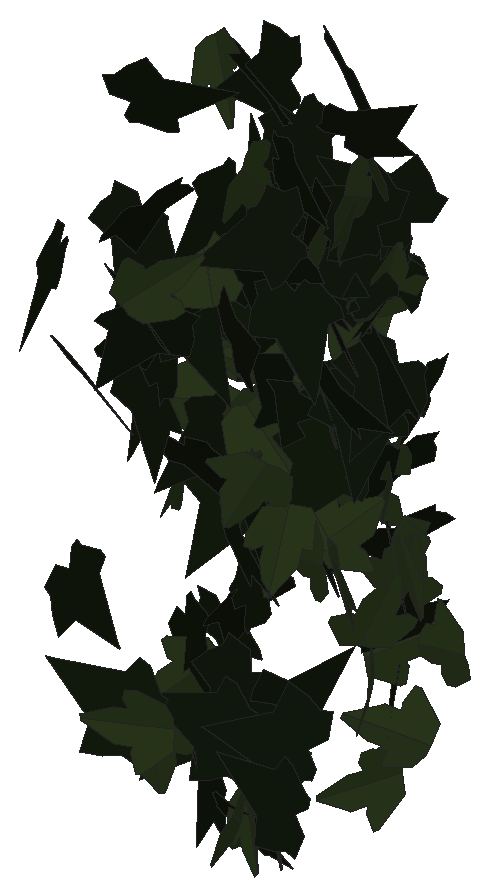
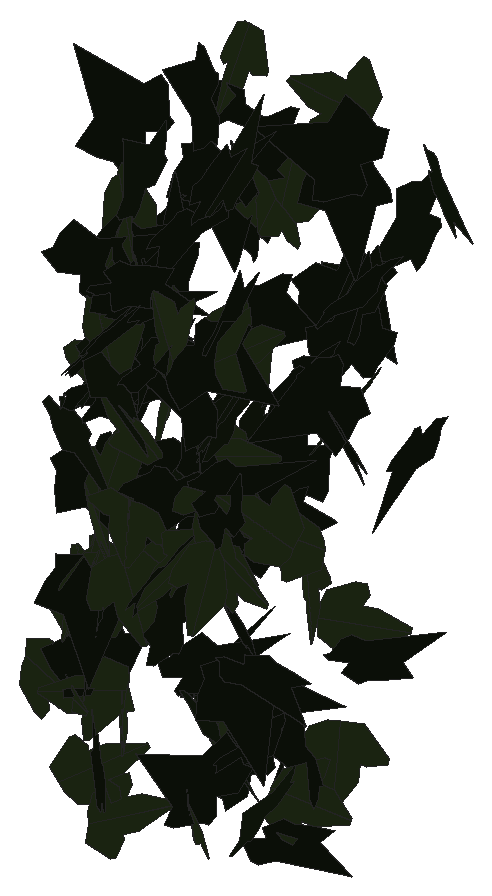
# SketchUp Ruby script. Lengths in inches.
U = 1.inch
M = Sketchup.active_model
def pt(a) = Geom::Point3d.new(a.map { |v| v * U })
def face(e, loops, mat)
  f = e.add_face(loops[0].map { |a| pt(a) })
  loops[1..].each { |l| e.add_face(l.map { |a| pt(a) }).erase! }
  f.material = f.back_material = mat if mat
  f
end
# faces: each face lists its corners as indices into pts; further lists are holes
def faces(e, pts, list, mat = nil) = list.each { |f| face(e, (f[0].is_a?(Array) ? f : [f]).map { |l| l.map { |i| pts[i] } }, mat) }
# xy, xz, yz: faces in a plane at the given z, y or x. An outline is a flat list of corners, or four numbers for a rectangle; further outlines are holes
def ring(l) = l.size == 4 ? [[l[0], l[1]], [l[2], l[1]], [l[2], l[3]], [l[0], l[3]]] : l.each_slice(2).to_a
def flat(e, list, mat, &to3) = list.each { |f| face(e, (f[0].is_a?(Array) ? f : [f]).map { |l| ring(l).map { |u, v| to3.(u, v) } }, mat) }
def xy(e, z, list, mat = nil) = flat(e, list, mat) { |x, y| [x, y, z] }
def xz(e, y, list, mat = nil) = flat(e, list, mat) { |x, z| [x, y, z] }
def yz(e, x, list, mat = nil) = flat(e, list, mat) { |y, z| [x, y, z] }
def lines(e, pts, list) = list.each { |a, b| e.add_line(pt(pts[a]), pt(pts[b])) }
# prism: a flat outline (further loops are holes) pulled along v
def prism(e, loops, v, mat = nil)
  f = face(e, loops, mat); d = Geom::Vector3d.new(v.map { |x| x * U })
  f.pushpull(f.normal.samedirection?(d) ? d.length : -d.length)
end
def box(e, o, s, mat = nil) = prism(e, [[o, [o[0] + s[0], o[1], o[2]], [o[0] + s[0], o[1] + s[1], o[2]], [o[0], o[1] + s[1], o[2]]]], [0, 0, s[2]], mat)
def at(x, y, z, deg = 0) = Geom::Transformation.translation(pt([x, y, z])) * Geom::Transformation.rotation(ORIGIN, Z_AXIS, deg.degrees)
def axes(o, x, y, z) = Geom::Transformation.new([*x, 0, *y, 0, *z, 0, *pt(o).to_a, 1])
def part(name) = M.definitions.add(name)
# library, detail: a bought-in or finely detailed component or shape, given as its bounding box
def library(name, o, s) = part(name).tap { |d| box(d.entities, o, s) }
def detail(e, o, s) = box(e.add_group.entities, o, s)
def put(e, d, t, mat = nil) = e.add_instance(d, t).tap { |i| i.material = mat if mat }
def group(e, t, mat = nil) = e.add_group.tap { |g| g.transformation = t; g.material = mat if mat }.entities
root = M.entities
M.materials.add("efeu1").color = [18, 25, 13]
M.materials.add("efeu2").color = [43, 57, 29]
c1 = part("ivyleaf_10")
p = [[0,0.5,-0.03],[-0.0625,2.02,-0.43],[-0.19,2.01,-0.46],[-0.54,1.05,-0.29],[-0.52,0.625,-0.18],[-0.83,0.76,-0.28],
  [-1.16,0.64,-0.33],[-1.15,0.33,-0.24],[-0.77,-0.39,0.02],[-0.3,-0.51,0.16],[0.04,-0.48,0.23],[-0.02,2.01,-0.4375],
  [-0.06,2.01,-0.43],[0.04,-0.49,0.23],[0.67,-0.49,0.14],[1.38,0.36,-0.2],[1.375,0.51,-0.24],[0.81,0.65,-0.19],
  [0.62,0.59,-0.15],[0.6,1.09,-0.28],[0.5,1.23,-0.31]]
faces(c1.entities,p,[[0,1,2,3,4,5,6,7,8,9,10],[11,12,0,13,14,15,16,17,18,19,20]],"efeu2")
c2 = part("ivyleaf_9")
p = [[1.54,2.16,1.25],[1.36,2.04,1.19],[-0.21,0.99,0.68],[-0.71,1.11,0.82],[-0.85,0.86,0.67],[-0.8,0.17,0.21],
  [-0.9,-0.01,0.1],[-0.67,-0.16,-0.02],[-0.08,-0.08,-0.05],[-0.03,-0.6,-0.4],[0.65,-0.88,-0.66],[0.83,-0.6,-0.49],
  [1.29,-0.42,-0.43],[1.8125,-0.07,-0.26],[1.21,0.44,0.15]]
faces(c2.entities,p,[[0,1,2,3,4,5,6,7,8,9,10,11,12,13,14]],"efeu1")
put(root,c1,axes([42.16,220.89,223.9],[-0.10723,-0.21957,0.43622],[-0.13695,-0.41518,-0.24264],[0.46877,-0.17151,0.0289]))
put(root,c1,axes([41.72,221.64,228.34],[-0.16814,-0.10366,0.45933],[0.43271,0.15836,0.19414],[-0.18573,0.46279,0.03646]))
put(root,c2,axes([42.16,221.76,226.26],[-0.45168,-0.20723,-0.05511],[0.04948,0.02431,-0.49695],[0.20865,-0.45438,-0.00146]))
put(root,c2,axes([41.99,219.8,231.16],[-0.0642,-0.47503,0.1422],[-0.0119,-0.14187,-0.4793],[0.49572,-0.06493,0.00691]))
put(root,c2,axes([41.85,221.79,224.1],[0.15319,-0.43883,0.18429],[0.09058,-0.16319,-0.46386],[0.46726,0.1755,0.0295]))
put(root,c1,axes([42.21,220.375,227.17],[0.15073,-0.43147,-0.20276],[-0.05057,0.19698,-0.45677],[0.47405,0.1582,0.01574]))
put(root,c2,axes([42.33,221.05,223.25],[-0.40647,-0.26211,0.12679],[-0.10699,-0.06804,-0.48366],[0.2708,-0.42032,-0.00078]))
put(root,c1,axes([41.84,220.93,227.88],[0.07247,-0.04418,-0.49274],[0.49418,-0.01688,0.07419],[-0.02319,-0.49776,0.04122]))
put(root,c2,axes([42.32,219.79,229.14],[-0.4026,0.01808,-0.29595],[0.29421,-0.03753,-0.40253],[-0.03677,-0.49826,0.01958]))
put(root,c2,axes([42.04,220.7,224.61],[-0.05356,-0.08047,-0.49057],[0.49466,0.04046,-0.06064],[0.04945,-0.49182,0.07527]))
put(root,c2,axes([42.37,217.51,231.82],[-0.35801,0.11658,-0.32899],[0.30532,-0.12376,-0.37612],[-0.16913,-0.4702,0.01742]))
put(root,c2,axes([42.27,219.74,229.59],[-0.0324,0.15923,-0.47286],[-0.06682,0.4682,0.16224],[0.49446,0.0737,-0.00906]))
put(root,c1,axes([42.09,221.24,233.1],[0.37263,-0.06917,0.32614],[0.31849,-0.07075,-0.37889],[0.09856,0.49011,-0.00866]))
put(root,c2,axes([42.7,221.87,228.81],[-0.16939,-0.36803,-0.29302],[-0.10718,-0.27305,0.40492],[-0.45806,0.19999,0.01361]))
put(root,c2,axes([42.04,219.61,233.0625],[0.18619,-0.02696,0.46325],[0.46375,-0.00683,-0.18679],[0.0164,0.49923,0.02246]))
put(root,c1,axes([42.81,221.48,227.49],[-0.0512,0.08277,0.49044],[-0.49606,0.02735,-0.0564],[-0.03616,-0.49234,0.07932]))
put(root,c2,axes([42.46,219.17,229.71],[0.21494,0.26282,0.36705],[-0.28836,-0.23286,0.33559],[0.34735,-0.35595,0.05147]))
put(root,c2,axes([42.58,220.79,227.79],[0.06705,-0.11388,-0.48222],[0.18822,-0.44429,0.13109],[-0.45834,-0.1991,-0.01671]))
put(root,c1,axes([42.625,221.53,230.71],[-0.01432,-0.00025,0.49979],[0.06894,-0.49522,0.00173],[0.49502,0.06897,0.01422]))
put(root,c1,axes([42.73,219.13,223.78],[-0.40536,-0.29201,-0.02033],[0.01689,0.01133,-0.49959],[0.29223,-0.40571,0.00068]))
put(root,c2,axes([42.48,219.32,228.91],[0.09118,-0.45663,0.18215],[0.05367,-0.1749,-0.46533],[0.48868,0.10441,0.01712]))
put(root,c2,axes([43.06,218.37,224.53],[-0.30083,-0.34643,-0.19872],[-0.13092,-0.1495,0.45881],[-0.37731,0.32808,-0.00076]))
put(root,c2,axes([42.58,220.02,229.87],[0.17465,-0.41391,-0.2195],[-0.05954,0.21274,-0.44855],[0.46471,0.18282,0.02502]))
put(root,c2,axes([42.4375,219,230.37],[0.149,-0.26705,0.39558],[0.23865,-0.3172,-0.30403],[0.41333,0.27941,0.03294]))
put(root,c2,axes([42.94,218.66,232.18],[-0.00362,0.49386,-0.07801],[0.00375,-0.07799,-0.49387],[-0.49997,-0.00416,-0.00313]))
put(root,c2,axes([42.99,221.79,230.85],[-0.01021,0.11717,-0.48597],[-0.04985,-0.48389,-0.11562],[-0.4974,0.04609,0.02157]))
put(root,c2,axes([42.58,221.75,228.32],[-0.05286,-0.01465,0.49698],[0.24206,-0.43731,0.01286],[0.4343,0.24196,0.05333]))
put(root,c2,axes([43.01,221.2,230.84],[-0.09319,-0.33968,0.35487],[0.08018,0.34584,0.35209],[-0.48465,0.12253,-0.00998]))
put(root,c2,axes([43.05,220.8,225.35],[-0.03421,0.46956,-0.16835],[0.01304,-0.16785,-0.47081],[-0.49866,-0.0366,-0.00076]))
put(root,c1,axes([42.91,221.58,227.52],[-0.27142,-0.38919,-0.15768],[0.08228,0.13482,-0.4744],[0.41178,-0.28347,-0.00914]))
put(root,c2,axes([43.1,218.63,230.54],[0.05978,0.27217,-0.41515],[-0.10421,-0.40195,-0.27852],[-0.48535,0.11982,0.00867]))
put(root,c2,axes([42.73,221.33,229.69],[0.25191,-0.37952,0.20618],[0.11234,-0.17289,-0.45551],[0.41704,0.27582,-0.00183]))
put(root,c2,axes([43.1,220.5,230.76],[-0.04248,0.00404,-0.49818],[0.18611,-0.46366,-0.01963],[-0.46212,-0.1871,0.03789]))
put(root,c2,axes([43.13,221.47,232.96],[-0.10812,-0.11905,0.47343],[-0.22419,-0.41863,-0.15647],[0.43364,-0.24612,0.03715]))
put(root,c2,axes([42.88,221.45,229.6],[0.01826,-0.35377,0.35287],[0.05145,-0.34989,-0.35345],[0.49701,0.04921,0.02362]))
put(root,c2,axes([43,221.2,232.93],[0.35529,-0.34938,-0.04123],[0.02979,-0.02852,0.4983],[-0.35055,-0.35654,0.00055]))
put(root,c1,axes([43.41,221.05,228.6875],[0.08757,0.08342,0.48515],[-0.40331,-0.27039,0.11929],[0.28227,-0.41222,0.01993]))
put(root,c2,axes([43.03,216.99,227.33],[0.19606,-0.28001,-0.36491],[-0.20991,0.29849,-0.34182],[0.40927,0.28723,-0.00051]))
put(root,c1,axes([43.2,221.0625,228.29],[-0.37493,-0.31752,-0.09277],[0.06942,0.06157,-0.49131],[0.32343,-0.3813,-0.00208]))
put(root,c2,axes([43.16,220.62,224.1875],[-0.14955,-0.43252,0.20139],[-0.07322,-0.18775,-0.45759],[0.47146,-0.16636,-0.00719]))
put(root,c2,axes([43.11,219.38,228.2],[0.47409,0.12482,-0.09829],[-0.09463,-0.02665,-0.49024],[-0.12762,0.48344,-0.00165]))
put(root,c2,axes([43,216.91,230.72],[0.47382,-0.15425,-0.04129],[-0.03886,0.01399,-0.49829],[0.15488,0.47541,0.00127]))
put(root,c1,axes([43.7,217.91,224.77],[0.03378,-0.00147,-0.49886],[-0.49438,-0.06692,-0.03328],[-0.06667,0.4955,-0.00597]))
put(root,c1,axes([43.07,220.8125,228.02],[0.34324,0.15882,0.32705],[0.28602,0.1597,-0.37774],[-0.22445,0.4464,0.01878]))
put(root,c2,axes([43.05,221.58,230.05],[0.14138,0.0096,-0.4795],[0.46701,0.11103,0.13992],[0.10916,-0.48742,0.02243]))
put(root,c1,axes([43.24,222.02,230.87],[-0.23636,-0.04739,0.43805],[0.41521,-0.19028,0.20345],[0.14742,0.45994,0.12931]))
put(root,c1,axes([43.55,221.31,227.25],[-0.02991,0.17392,0.46782],[-0.06606,0.46316,-0.17641],[-0.49471,-0.07236,-0.00473]))
put(root,c2,axes([43.56,220.9375,228.53],[0.07398,0.14242,0.47354],[-0.23462,-0.41138,0.16038],[0.43529,-0.24594,0.00596]))
put(root,c2,axes([43.45,220.24,225.6],[-0.18153,0.32813,0.33072],[0.1644,-0.28699,0.37498],[0.43591,0.24489,-0.00369]))
put(root,c2,axes([43.44,221.3125,232.51],[0.1054,-0.42144,-0.24755],[-0.05742,0.2408,-0.43441],[0.48538,0.12,0.00236]))
put(root,c2,axes([44.02,219.23,224.21],[-0.29608,-0.15036,-0.37381],[-0.3271,-0.18116,0.33195],[-0.23526,0.44111,0.00891]))
put(root,c2,axes([43.47,220.85,223.45],[-0.06705,-0.03198,0.49445],[0.42209,0.25765,0.0739],[-0.25951,0.42731,-0.00755]))
put(root,c2,axes([43.4375,219.47,223.29],[0.13348,-0.11232,-0.46858],[0.40025,-0.24488,0.17272],[-0.26829,-0.42121,0.02454]))
put(root,c2,axes([43.34,221.75,226.52],[0.28331,-0.26966,0.31148],[0.2306,-0.20947,-0.39108],[0.34141,0.36525,0.00568]))
put(root,c2,axes([43.57,221.77,227.29],[0.18538,-0.44932,-0.11725],[-0.05094,0.10581,-0.48601],[0.46156,0.19214,-0.00655]))
put(root,c2,axes([43.6,221.49,228.43],[-0.10632,-0.3165,-0.37219],[0.11653,0.35348,-0.33388],[0.47447,-0.15774,-0.0014]))
put(root,c1,axes([43.61,221.11,223.26],[0.31392,-0.22476,0.31771],[0.26708,-0.17246,-0.38591],[0.28305,0.412,0.01178]))
put(root,c1,axes([43.79,219.91,227.86],[0.25861,-0.39216,0.17127],[0.09371,-0.14336,-0.46975],[0.41754,0.27506,-0.00065]))
put(root,c2,axes([43.98,219.99,227.34],[0.31656,0.16167,-0.35165],[-0.31677,-0.15279,-0.3554],[-0.22237,0.44779,0.00569]))
put(root,c2,axes([43.71,220.98,228.54],[-0.04861,-0.3371,0.36606],[0.09802,-0.36709,-0.32502],[0.48788,0.04017,0.10177]))
put(root,c2,axes([43.93,219.33,232.53],[-0.01005,0.03183,-0.49888],[0.20085,-0.45668,-0.03318],[-0.45778,-0.20106,-0.00361]))
put(root,c2,axes([43.98,221.69,230.23],[-0.18723,-0.34282,0.31212],[-0.1609,-0.26765,-0.39048],[0.43481,-0.24666,-0.0101]))
put(root,c1,axes([43.98,218.74,231.26],[0.27958,0.41352,0.02894],[-0.02242,-0.01977,0.49911],[0.41393,-0.28037,0.00749]))
put(root,c2,axes([43.75,221.98,233.14],[0.11988,-0.29796,0.38321],[0.16616,-0.34569,-0.32076],[0.45609,0.20426,0.01614]))
put(root,c1,axes([44.33,221.69,226.9],[-0.41013,-0.21321,0.19061],[-0.17064,-0.08498,-0.46223],[0.2295,-0.44421,-0.00306]))
put(root,c2,axes([44.39,221.77,231.33],[-0.40798,-0.20721,0.20153],[-0.1836,-0.08349,-0.45752],[0.22325,-0.44732,-0.00796]))
put(root,c1,axes([44.17,220.98,231.15],[0.18198,-0.43842,0.15707],[0.079,-0.13713,-0.47429],[0.45896,0.19744,0.01936]))
put(root,c1,axes([44.07,221.86,228.01],[0.48043,0.07048,0.11923],[0.11616,0.02937,-0.48543],[-0.07543,0.49414,0.01185]))
put(root,c1,axes([43.93,221.76,229.02],[0.35779,-0.15892,-0.31101],[0.31852,-0.03419,0.3839],[-0.14328,-0.47284,0.07677]))
put(root,c2,axes([43.9375,220.91,226.6],[0.18479,-0.31985,0.33697],[0.16577,-0.29338,-0.36939],[0.43402,0.24823,-0.00239]))
put(root,c2,axes([44.22,220.78,231.02],[0.05082,0.33905,0.36395],[-0.17839,-0.32908,0.33148],[0.46432,-0.16354,0.08752]))
put(root,c1,axes([44.19,216.98,231.96],[-0.1472,-0.25667,0.40305],[0.18166,0.36002,0.29561],[-0.44196,0.23346,-0.01274]))
put(root,c2,axes([44.7,221.36,231.35],[-0.07545,-0.00431,0.49426],[-0.46376,-0.17235,-0.0723],[0.17099,-0.46934,0.02201]))
put(root,c1,axes([44.49,218.67,223.34],[0.00043,-0.3719,-0.3342],[-0.01193,0.3341,-0.3718],[0.49986,0.00829,-0.00859]))
put(root,c2,axes([44.67,221.74,230.11],[-0.30252,0.3908,-0.07586],[0.04547,-0.06073,-0.49421],[-0.39549,-0.30592,0.0012]))
put(root,c2,axes([44.72,221.47,230.63],[-0.27399,-0.09365,0.40763],[-0.33864,-0.23632,-0.28191],[0.24547,-0.43056,0.06607]))
put(root,c1,axes([44.76,221.28,232.4],[-0.26068,0.10688,0.41307],[-0.38124,0.15902,-0.28173],[-0.19159,-0.46183,-0.00141]))
put(root,c1,axes([44.51,220.45,229.2],[-0.34323,0.35701,0.06882],[-0.04765,0.04966,-0.49524],[-0.36045,-0.34652,-0.00007]))
put(root,c2,axes([44.17,219.21,222.86],[0.45747,-0.03244,-0.19918],[0.19901,-0.00923,0.45859],[-0.03343,-0.49886,0.00446]))
put(root,c2,axes([44.48,222.21,230.45],[-0.15312,-0.34672,0.3261],[-0.0523,-0.32823,-0.37354],[0.4731,-0.1485,0.06425]))
put(root,c2,axes([44.65,220.7,228.16],[-0.39448,-0.30496,0.03719],[-0.02388,-0.0299,-0.49853],[0.30629,-0.3951,0.00903]))
put(root,c1,axes([44.62,221.02,231.72],[0.19759,-0.45555,-0.05858],[-0.0202,0.0551,-0.49654],[0.45886,0.1986,0.00337]))
put(root,c2,axes([44.58,222.19,230.41],[-0.19483,-0.25784,0.38152],[-0.07477,-0.39105,-0.30247],[0.45437,-0.17492,0.11382]))
put(root,c2,axes([44.69,219.07,231.89],[0.25463,0.32198,-0.28547],[-0.16774,-0.23119,-0.41038],[-0.39627,0.30476,-0.00972]))
put(root,c2,axes([44.93,221.78,231.32],[-0.01466,0.04556,0.4977],[-0.49932,0.0201,-0.01655],[-0.02152,-0.49751,0.04491]))
put(root,c2,axes([44.5,218.56,227.81],[0.39804,-0.16096,-0.25623],[-0.23019,0.11373,-0.42904],[0.1964,0.45952,0.01644]))
put(root,c2,axes([44.68,220.45,230.33],[0.34433,-0.02987,-0.36131],[-0.35693,0.05942,-0.34507],[0.06355,0.49556,0.0196]))
put(root,c2,axes([44.94,219.3,223.55],[-0.38076,0.31918,0.05611],[-0.04216,0.03705,-0.49684],[-0.32132,-0.38308,-0.0013]))
put(root,c1,axes([44.69,220.875,232.02],[-0.00691,-0.25767,-0.42844],[0.03943,0.42686,-0.25736],[0.49839,-0.03734,0.01442]))
put(root,c2,axes([44.96,219.54,224.18],[-0.18216,0.00429,0.46562],[-0.41144,-0.23558,-0.1588],[0.21802,-0.441,0.08936]))
put(root,c2,axes([44.52,221.95,223.62],[-0.00932,0.20426,0.45628],[0.02714,-0.45548,0.20445],[0.49918,0.02857,-0.0026]))
put(root,c1,axes([44.875,221.42,222.85],[0.02812,0.03381,-0.49806],[-0.30463,-0.39404,-0.04395],[-0.39549,0.30592,-0.00156]))
put(root,c1,axes([44.69,221.59,230.01],[-0.12857,-0.4825,0.02581],[0.0067,0.02493,0.49933],[-0.48314,0.12875,0.00005]))
put(root,c2,axes([44.88,221.64,226.59],[0.10558,0.48309,-0.07399],[-0.01951,-0.07147,-0.49448],[-0.48834,0.1073,0.00376]))
put(root,c1,axes([44.48,218.83,223.47],[0.27851,-0.11157,0.39998],[0.3719,-0.14723,-0.30003],[0.18472,0.46463,0.00097]))
put(root,c1,axes([44.92,221.28,227.82],[-0.48015,-0.07379,-0.11836],[-0.11338,-0.04066,0.48528],[-0.08124,0.49285,0.02232]))
put(root,c1,axes([44.82,218.49,233.43],[0.00361,-0.38525,-0.3187],[0.0683,0.31611,-0.38133],[0.4953,-0.04078,0.0549]))
put(root,c1,axes([44.51,220.67,226.77],[0.33868,0.01034,-0.36768],[0.36634,0.03541,0.33844],[0.03303,-0.49864,0.01641]))
put(root,c2,axes([44.94,221.49,226.31],[0.24268,-0.06362,-0.43251],[-0.41774,0.11205,-0.25087],[0.12884,0.48311,0.00123]))
put(root,c2,axes([44.55,218.55,230.67],[0.0237,-0.03389,0.49829],[0.21473,-0.4497,-0.0408],[0.45092,0.21593,-0.00677]))
put(root,c1,axes([44.81,219.34,227.67],[0.25109,0.40636,-0.14775],[-0.07108,-0.12974,-0.47761],[-0.4265,0.26085,-0.00738]))
put(root,c1,axes([44.71,219.1,223.58],[-0.27432,0.3044,-0.28651],[0.16137,-0.23902,-0.40845],[-0.38563,-0.31656,0.0329]))
put(root,c1,axes([45.21,219.54,227.11],[-0.11581,0.08816,0.47835],[-0.47124,0.10148,-0.1328],[-0.1205,-0.48159,0.05959]))
put(root,c1,axes([45.03,220.87,224.65],[0.177,-0.3367,-0.32451],[-0.12193,0.30174,-0.37958],[0.45145,0.21351,0.02471]))
put(root,c1,axes([45.14,218.37,228.96],[-0.35216,-0.25574,0.24614],[-0.1855,-0.163,-0.43476],[0.30261,-0.39753,0.01992]))
put(root,c1,axes([45.15,221.64,223.48],[0.11371,0.20407,0.44207],[-0.22772,-0.37897,0.23351],[0.43036,-0.25444,0.00675]))
put(root,c1,axes([44.9,221.62,227.82],[0.23984,-0.41057,0.15463],[0.10063,-0.12005,-0.47483],[0.42703,0.25889,0.02504]))
put(root,c2,axes([45.32,218.73,232.57],[-0.45145,0.01551,0.21437],[-0.21409,0.0115,-0.4517],[-0.01894,-0.49963,-0.00374]))
put(root,c1,axes([44.78,221.43,224.82],[0.04935,0.05704,-0.49428],[0.34503,0.35395,0.07529],[0.35849,-0.34852,-0.00443]))
put(root,c2,axes([44.63,219.49,233.08],[0.16294,-0.06358,-0.46841],[0.47229,0.04265,0.1585],[0.0198,-0.4941,0.07396]))
put(root,c2,axes([45.24,221.2,228.1],[-0.07349,0.4132,-0.27178],[-0.00234,-0.27505,-0.41754],[-0.49456,-0.0601,0.04236]))
put(root,c2,axes([44.94,221.43,225.09],[0.31543,0.29199,0.25543],[-0.19031,-0.17041,0.42982],[0.33806,-0.36837,0.00363]))
put(root,c1,axes([45.04,221.52,225.87],[-0.44976,-0.18277,0.11965],[0.12073,0.02026,0.48478],[-0.18206,0.46496,0.0259]))
put(root,c2,axes([45.04,220.79,229.05],[-0.10308,-0.4889,-0.01866],[0.00375,0.01828,-0.49965],[0.48925,-0.10315,-0.0001]))
put(root,c2,axes([45.3125,218.84,223.62],[-0.01685,-0.49942,-0.01706],[0.00042,-0.01708,0.49971],[-0.49972,0.01682,0.00099]))
put(root,c2,axes([45.15,221.27,229.34],[-0.21491,-0.44009,0.10067],[-0.04553,-0.0898,-0.48976],[0.44916,-0.21967,-0.00147]))
put(root,c2,axes([44.84,220.68,233.06],[0.43041,0.21914,-0.12932],[0.09971,0.08855,0.48189],[0.23411,-0.44061,0.03252]))
put(root,c1,axes([45.19,221.4,226.53],[-0.13666,0.43399,0.20732],[-0.0755,0.19349,-0.45482],[-0.475,-0.15561,0.01265]))
put(root,c2,axes([44.78,220.25,229.24],[0.21063,-0.17565,0.41807],[0.32892,-0.25815,-0.27418],[0.31216,0.39052,0.0068]))
put(root,c2,axes([45.4375,221.58,228.88],[-0.35653,0.34927,-0.02992],[0.02148,-0.02083,-0.4991],[-0.34989,-0.35718,-0.00015]))
put(root,c2,axes([45.07,219.23,231.29],[0.00491,-0.47281,-0.16256],[0.0037,0.1626,-0.47281],[0.49996,0.00344,0.00509]))
put(root,c1,axes([45.33,221.27,226.58],[-0.17831,0.46667,0.02053],[-0.0043,0.02033,-0.49957],[-0.4671,-0.17833,-0.00324]))
put(root,c1,axes([45.29,220.53,225.64],[-0.23097,-0.42274,0.13396],[0.06825,0.11536,0.4817],[-0.43817,0.24081,0.00441]))
put(root,c1,axes([45.76,221.78,224.97],[-0.10278,0.02109,0.48887],[-0.48821,-0.03801,-0.101],[0.03291,-0.49811,0.02841]))
put(root,c1,axes([45.42,219.6875,227.0625],[-0.36922,0.32949,0.07148],[-0.05112,0.05007,-0.49485],[-0.33326,-0.37273,-0.00329]))
put(root,c2,axes([45.17,221.2,229.37],[0.03105,-0.33685,0.36819],[0.09905,-0.3574,-0.33534],[0.48911,0.09377,0.04453]))
